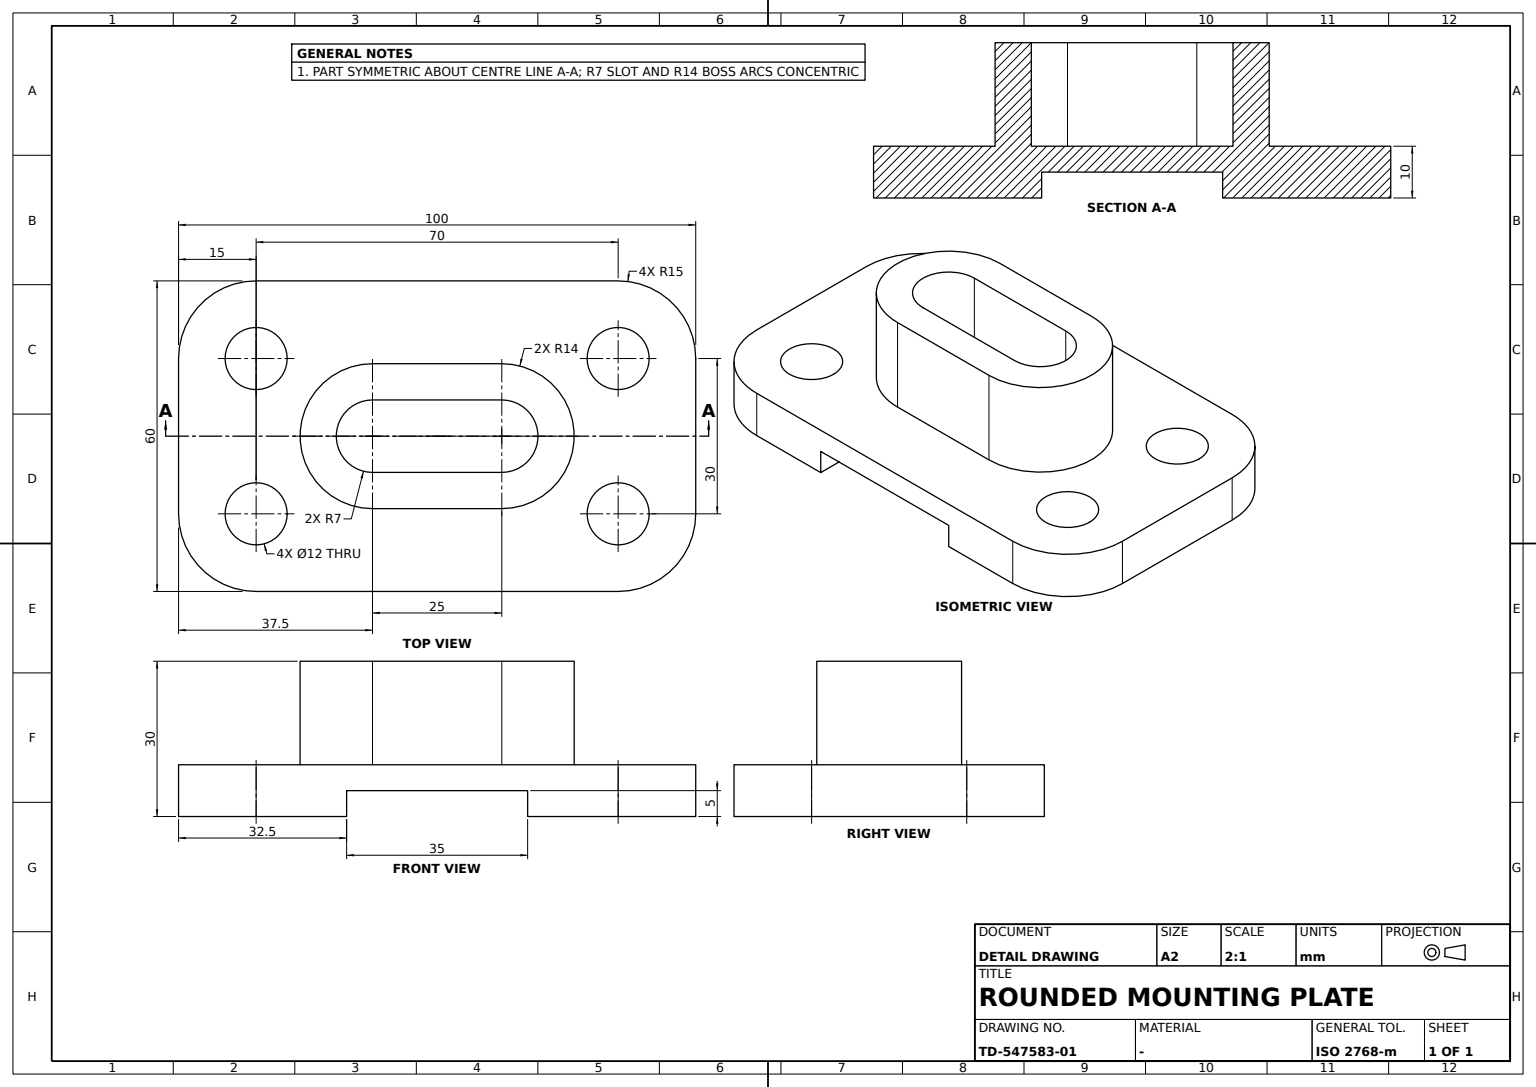
ISO-10303-21;
HEADER;
FILE_DESCRIPTION((''),'2;1');
FILE_NAME('','',(''),(''),'','','');
FILE_SCHEMA(('AUTOMOTIVE_DESIGN'));
ENDSEC;
DATA;
#1=APPLICATION_CONTEXT('');
#2=PRODUCT_CONTEXT('',#1,'mechanical');
#3=PRODUCT('','','',(#2));
#4=PRODUCT_DEFINITION_FORMATION('','',#3);
#5=PRODUCT_DEFINITION_CONTEXT('',#1,'design');
#6=PRODUCT_DEFINITION('','',#4,#5);
#7=PRODUCT_DEFINITION_SHAPE('','',#6);
#8=(LENGTH_UNIT()NAMED_UNIT(*)SI_UNIT(.MILLI.,.METRE.));
#9=(NAMED_UNIT(*)PLANE_ANGLE_UNIT()SI_UNIT($,.RADIAN.));
#10=(NAMED_UNIT(*)SI_UNIT($,.STERADIAN.)SOLID_ANGLE_UNIT());
#11=UNCERTAINTY_MEASURE_WITH_UNIT(LENGTH_MEASURE(0.005),#8,'distance_accuracy_value','');
#12=(GEOMETRIC_REPRESENTATION_CONTEXT(3)GLOBAL_UNCERTAINTY_ASSIGNED_CONTEXT((#11))GLOBAL_UNIT_ASSIGNED_CONTEXT((#8,#9,#10))REPRESENTATION_CONTEXT('',''));
#13=CARTESIAN_POINT('',(17.5,30.,0.));
#14=VERTEX_POINT('',#13);
#15=CARTESIAN_POINT('',(17.5,-30.,0.));
#16=VERTEX_POINT('',#15);
#17=CARTESIAN_POINT('',(17.5,0.,0.));
#18=DIRECTION('',(0.,-1.,0.));
#19=VECTOR('',#18,1000.);
#20=LINE('',#17,#19);
#21=EDGE_CURVE('',#14,#16,#20,.T.);
#22=ORIENTED_EDGE('',*,*,#21,.T.);
#23=CARTESIAN_POINT('',(17.5,-30.,5.));
#24=VERTEX_POINT('',#23);
#25=DIRECTION('',(0.,0.,1.));
#26=VECTOR('',#25,1000.);
#27=LINE('',#15,#26);
#28=EDGE_CURVE('',#16,#24,#27,.T.);
#29=ORIENTED_EDGE('',*,*,#28,.T.);
#30=CARTESIAN_POINT('',(17.5,30.,5.));
#31=VERTEX_POINT('',#30);
#32=LINE('',#30,#19);
#33=EDGE_CURVE('',#31,#24,#32,.T.);
#34=ORIENTED_EDGE('',*,*,#33,.F.);
#35=DIRECTION('',(0.,0.,-1.));
#36=VECTOR('',#35,1000.);
#37=LINE('',#13,#36);
#38=EDGE_CURVE('',#31,#14,#37,.T.);
#39=ORIENTED_EDGE('',*,*,#38,.T.);
#40=EDGE_LOOP('',(#22,#29,#34,#39));
#41=FACE_BOUND('',#40,.T.);
#42=DIRECTION('',(-1.,0.,0.));
#43=AXIS2_PLACEMENT_3D('',#30,#42,#35);
#44=PLANE('',#43);
#45=ADVANCED_FACE('',(#41),#44,.T.);
#46=CARTESIAN_POINT('',(-29.,15.,0.));
#47=VERTEX_POINT('',#46);
#48=CARTESIAN_POINT('',(-35.,15.,0.));
#49=DIRECTION('',(1.,0.,0.));
#50=AXIS2_PLACEMENT_3D('',#48,#25,#49);
#51=CIRCLE('',#50,6.);
#52=EDGE_CURVE('',#47,#47,#51,.T.);
#53=ORIENTED_EDGE('',*,*,#52,.T.);
#54=EDGE_LOOP('',(#53));
#55=FACE_BOUND('',#54,.T.);
#56=CARTESIAN_POINT('',(-50.,-15.,0.));
#57=VERTEX_POINT('',#56);
#58=CARTESIAN_POINT('',(-50.,15.,0.));
#59=VERTEX_POINT('',#58);
#60=CARTESIAN_POINT('',(-50.,0.,0.));
#61=DIRECTION('',(0.,1.,0.));
#62=VECTOR('',#61,1000.);
#63=LINE('',#60,#62);
#64=EDGE_CURVE('',#57,#59,#63,.T.);
#65=ORIENTED_EDGE('',*,*,#64,.T.);
#66=CARTESIAN_POINT('',(-35.,30.,0.));
#67=VERTEX_POINT('',#66);
#68=CIRCLE('',#50,15.);
#69=EDGE_CURVE('',#67,#59,#68,.T.);
#70=ORIENTED_EDGE('',*,*,#69,.F.);
#71=CARTESIAN_POINT('',(-17.5,30.,0.));
#72=VERTEX_POINT('',#71);
#73=CARTESIAN_POINT('',(0.,30.,0.));
#74=VECTOR('',#49,1000.);
#75=LINE('',#73,#74);
#76=EDGE_CURVE('',#67,#72,#75,.T.);
#77=ORIENTED_EDGE('',*,*,#76,.T.);
#78=CARTESIAN_POINT('',(-17.5,-30.,0.));
#79=VERTEX_POINT('',#78);
#80=LINE('',#71,#19);
#81=EDGE_CURVE('',#72,#79,#80,.T.);
#82=ORIENTED_EDGE('',*,*,#81,.T.);
#83=CARTESIAN_POINT('',(-35.,-30.,0.));
#84=VERTEX_POINT('',#83);
#85=CARTESIAN_POINT('',(0.,-30.,0.));
#86=VECTOR('',#42,1000.);
#87=LINE('',#85,#86);
#88=EDGE_CURVE('',#79,#84,#87,.T.);
#89=ORIENTED_EDGE('',*,*,#88,.T.);
#90=CARTESIAN_POINT('',(-35.,-15.,0.));
#91=AXIS2_PLACEMENT_3D('',#90,#25,#49);
#92=CIRCLE('',#91,15.);
#93=EDGE_CURVE('',#57,#84,#92,.T.);
#94=ORIENTED_EDGE('',*,*,#93,.F.);
#95=EDGE_LOOP('',(#65,#70,#77,#82,#89,#94));
#96=FACE_BOUND('',#95,.T.);
#97=CARTESIAN_POINT('',(-29.,-15.,0.));
#98=VERTEX_POINT('',#97);
#99=CIRCLE('',#91,6.);
#100=EDGE_CURVE('',#98,#98,#99,.T.);
#101=ORIENTED_EDGE('',*,*,#100,.T.);
#102=EDGE_LOOP('',(#101));
#103=FACE_BOUND('',#102,.T.);
#104=CARTESIAN_POINT('',(0.,0.,0.));
#105=AXIS2_PLACEMENT_3D('',#104,#25,#49);
#106=PLANE('',#105);
#107=ADVANCED_FACE('',(#55,#96,#103),#106,.F.);
#108=ORIENTED_EDGE('',*,*,#100,.F.);
#109=EDGE_LOOP('',(#108));
#110=FACE_BOUND('',#109,.T.);
#111=CARTESIAN_POINT('',(-29.,-15.,10.));
#112=VERTEX_POINT('',#111);
#113=CARTESIAN_POINT('',(-35.,-15.,10.));
#114=AXIS2_PLACEMENT_3D('',#113,#25,#49);
#115=CIRCLE('',#114,6.);
#116=EDGE_CURVE('',#112,#112,#115,.T.);
#117=ORIENTED_EDGE('',*,*,#116,.T.);
#118=EDGE_LOOP('',(#117));
#119=FACE_BOUND('',#118,.T.);
#120=CARTESIAN_POINT('',(-35.,-15.,5.));
#121=AXIS2_PLACEMENT_3D('',#120,#25,#49);
#122=CYLINDRICAL_SURFACE('',#121,6.);
#123=ADVANCED_FACE('',(#110,#119),#122,.F.);
#124=CARTESIAN_POINT('',(12.5,-14.,30.));
#125=VERTEX_POINT('',#124);
#126=CARTESIAN_POINT('',(12.5,14.,30.));
#127=VERTEX_POINT('',#126);
#128=CARTESIAN_POINT('',(12.5,0.,30.));
#129=AXIS2_PLACEMENT_3D('',#128,#25,#49);
#130=CIRCLE('',#129,14.);
#131=EDGE_CURVE('',#125,#127,#130,.T.);
#132=ORIENTED_EDGE('',*,*,#131,.F.);
#133=CARTESIAN_POINT('',(12.5,-14.,10.));
#134=VERTEX_POINT('',#133);
#135=CARTESIAN_POINT('',(12.5,-14.,20.));
#136=LINE('',#135,#26);
#137=EDGE_CURVE('',#134,#125,#136,.T.);
#138=ORIENTED_EDGE('',*,*,#137,.F.);
#139=CARTESIAN_POINT('',(12.5,14.,10.));
#140=VERTEX_POINT('',#139);
#141=CARTESIAN_POINT('',(12.5,0.,10.));
#142=AXIS2_PLACEMENT_3D('',#141,#25,#49);
#143=CIRCLE('',#142,14.);
#144=EDGE_CURVE('',#134,#140,#143,.T.);
#145=ORIENTED_EDGE('',*,*,#144,.T.);
#146=CARTESIAN_POINT('',(12.5,14.,20.));
#147=LINE('',#146,#26);
#148=EDGE_CURVE('',#140,#127,#147,.T.);
#149=ORIENTED_EDGE('',*,*,#148,.T.);
#150=EDGE_LOOP('',(#132,#138,#145,#149));
#151=FACE_BOUND('',#150,.T.);
#152=CARTESIAN_POINT('',(12.5,0.,20.));
#153=AXIS2_PLACEMENT_3D('',#152,#25,#49);
#154=CYLINDRICAL_SURFACE('',#153,14.);
#155=ADVANCED_FACE('',(#151),#154,.T.);
#156=CARTESIAN_POINT('',(50.,15.,10.));
#157=VERTEX_POINT('',#156);
#158=CARTESIAN_POINT('',(50.,-15.,10.));
#159=VERTEX_POINT('',#158);
#160=CARTESIAN_POINT('',(50.,0.,10.));
#161=LINE('',#160,#19);
#162=EDGE_CURVE('',#157,#159,#161,.T.);
#163=ORIENTED_EDGE('',*,*,#162,.T.);
#164=CARTESIAN_POINT('',(50.,-15.,0.));
#165=VERTEX_POINT('',#164);
#166=CARTESIAN_POINT('',(50.,-15.,5.));
#167=LINE('',#166,#26);
#168=EDGE_CURVE('',#165,#159,#167,.T.);
#169=ORIENTED_EDGE('',*,*,#168,.F.);
#170=CARTESIAN_POINT('',(50.,15.,0.));
#171=VERTEX_POINT('',#170);
#172=CARTESIAN_POINT('',(50.,0.,0.));
#173=LINE('',#172,#19);
#174=EDGE_CURVE('',#171,#165,#173,.T.);
#175=ORIENTED_EDGE('',*,*,#174,.F.);
#176=CARTESIAN_POINT('',(50.,15.,5.));
#177=LINE('',#176,#26);
#178=EDGE_CURVE('',#171,#157,#177,.T.);
#179=ORIENTED_EDGE('',*,*,#178,.T.);
#180=EDGE_LOOP('',(#163,#169,#175,#179));
#181=FACE_BOUND('',#180,.T.);
#182=AXIS2_PLACEMENT_3D('',#170,#42,#18);
#183=PLANE('',#182);
#184=ADVANCED_FACE('',(#181),#183,.F.);
#185=CARTESIAN_POINT('',(-29.,15.,10.));
#186=VERTEX_POINT('',#185);
#187=CARTESIAN_POINT('',(-35.,15.,10.));
#188=AXIS2_PLACEMENT_3D('',#187,#25,#49);
#189=CIRCLE('',#188,6.);
#190=EDGE_CURVE('',#186,#186,#189,.T.);
#191=ORIENTED_EDGE('',*,*,#190,.F.);
#192=EDGE_LOOP('',(#191));
#193=FACE_BOUND('',#192,.T.);
#194=ORIENTED_EDGE('',*,*,#116,.F.);
#195=EDGE_LOOP('',(#194));
#196=FACE_BOUND('',#195,.T.);
#197=CARTESIAN_POINT('',(-50.,-15.,10.));
#198=VERTEX_POINT('',#197);
#199=CARTESIAN_POINT('',(-35.,-30.,10.));
#200=VERTEX_POINT('',#199);
#201=CIRCLE('',#114,15.);
#202=EDGE_CURVE('',#198,#200,#201,.T.);
#203=ORIENTED_EDGE('',*,*,#202,.T.);
#204=CARTESIAN_POINT('',(35.,-30.,10.));
#205=VERTEX_POINT('',#204);
#206=CARTESIAN_POINT('',(0.,-30.,10.));
#207=LINE('',#206,#86);
#208=EDGE_CURVE('',#205,#200,#207,.T.);
#209=ORIENTED_EDGE('',*,*,#208,.F.);
#210=CARTESIAN_POINT('',(35.,-15.,10.));
#211=AXIS2_PLACEMENT_3D('',#210,#25,#49);
#212=CIRCLE('',#211,15.);
#213=EDGE_CURVE('',#205,#159,#212,.T.);
#214=ORIENTED_EDGE('',*,*,#213,.T.);
#215=ORIENTED_EDGE('',*,*,#162,.F.);
#216=CARTESIAN_POINT('',(35.,30.,10.));
#217=VERTEX_POINT('',#216);
#218=CARTESIAN_POINT('',(35.,15.,10.));
#219=AXIS2_PLACEMENT_3D('',#218,#25,#49);
#220=CIRCLE('',#219,15.);
#221=EDGE_CURVE('',#157,#217,#220,.T.);
#222=ORIENTED_EDGE('',*,*,#221,.T.);
#223=CARTESIAN_POINT('',(-35.,30.,10.));
#224=VERTEX_POINT('',#223);
#225=CARTESIAN_POINT('',(0.,30.,10.));
#226=LINE('',#225,#74);
#227=EDGE_CURVE('',#224,#217,#226,.T.);
#228=ORIENTED_EDGE('',*,*,#227,.F.);
#229=CARTESIAN_POINT('',(-50.,15.,10.));
#230=VERTEX_POINT('',#229);
#231=CIRCLE('',#188,15.);
#232=EDGE_CURVE('',#224,#230,#231,.T.);
#233=ORIENTED_EDGE('',*,*,#232,.T.);
#234=CARTESIAN_POINT('',(-50.,0.,10.));
#235=LINE('',#234,#62);
#236=EDGE_CURVE('',#198,#230,#235,.T.);
#237=ORIENTED_EDGE('',*,*,#236,.F.);
#238=EDGE_LOOP('',(#203,#209,#214,#215,#222,#228,#233,#237));
#239=FACE_BOUND('',#238,.T.);
#240=CARTESIAN_POINT('',(-12.5,-14.,10.));
#241=VERTEX_POINT('',#240);
#242=CARTESIAN_POINT('',(0.,-14.,10.));
#243=LINE('',#242,#74);
#244=EDGE_CURVE('',#241,#134,#243,.T.);
#245=ORIENTED_EDGE('',*,*,#244,.F.);
#246=CARTESIAN_POINT('',(-12.5,14.,10.));
#247=VERTEX_POINT('',#246);
#248=CARTESIAN_POINT('',(-12.5,0.,10.));
#249=AXIS2_PLACEMENT_3D('',#248,#25,#49);
#250=CIRCLE('',#249,14.);
#251=EDGE_CURVE('',#247,#241,#250,.T.);
#252=ORIENTED_EDGE('',*,*,#251,.F.);
#253=CARTESIAN_POINT('',(0.,14.,10.));
#254=LINE('',#253,#74);
#255=EDGE_CURVE('',#247,#140,#254,.T.);
#256=ORIENTED_EDGE('',*,*,#255,.T.);
#257=ORIENTED_EDGE('',*,*,#144,.F.);
#258=EDGE_LOOP('',(#245,#252,#256,#257));
#259=FACE_BOUND('',#258,.T.);
#260=CARTESIAN_POINT('',(41.,15.,10.));
#261=VERTEX_POINT('',#260);
#262=CIRCLE('',#219,6.);
#263=EDGE_CURVE('',#261,#261,#262,.T.);
#264=ORIENTED_EDGE('',*,*,#263,.F.);
#265=EDGE_LOOP('',(#264));
#266=FACE_BOUND('',#265,.T.);
#267=CARTESIAN_POINT('',(41.,-15.,10.));
#268=VERTEX_POINT('',#267);
#269=CIRCLE('',#211,6.);
#270=EDGE_CURVE('',#268,#268,#269,.T.);
#271=ORIENTED_EDGE('',*,*,#270,.F.);
#272=EDGE_LOOP('',(#271));
#273=FACE_BOUND('',#272,.T.);
#274=CARTESIAN_POINT('',(0.,0.,10.));
#275=AXIS2_PLACEMENT_3D('',#274,#25,#49);
#276=PLANE('',#275);
#277=ADVANCED_FACE('',(#193,#196,#239,#259,#266,#273),#276,.T.);
#278=CARTESIAN_POINT('',(-12.5,-14.,30.));
#279=VERTEX_POINT('',#278);
#280=CARTESIAN_POINT('',(0.,-14.,30.));
#281=LINE('',#280,#74);
#282=EDGE_CURVE('',#279,#125,#281,.T.);
#283=ORIENTED_EDGE('',*,*,#282,.F.);
#284=CARTESIAN_POINT('',(-12.5,-14.,20.));
#285=LINE('',#284,#26);
#286=EDGE_CURVE('',#241,#279,#285,.T.);
#287=ORIENTED_EDGE('',*,*,#286,.F.);
#288=ORIENTED_EDGE('',*,*,#244,.T.);
#289=ORIENTED_EDGE('',*,*,#137,.T.);
#290=EDGE_LOOP('',(#283,#287,#288,#289));
#291=FACE_BOUND('',#290,.T.);
#292=AXIS2_PLACEMENT_3D('',#240,#18,#49);
#293=PLANE('',#292);
#294=ADVANCED_FACE('',(#291),#293,.T.);
#295=ORIENTED_EDGE('',*,*,#251,.T.);
#296=ORIENTED_EDGE('',*,*,#286,.T.);
#297=CARTESIAN_POINT('',(-12.5,14.,30.));
#298=VERTEX_POINT('',#297);
#299=CARTESIAN_POINT('',(-12.5,0.,30.));
#300=AXIS2_PLACEMENT_3D('',#299,#25,#49);
#301=CIRCLE('',#300,14.);
#302=EDGE_CURVE('',#298,#279,#301,.T.);
#303=ORIENTED_EDGE('',*,*,#302,.F.);
#304=CARTESIAN_POINT('',(-12.5,14.,20.));
#305=LINE('',#304,#26);
#306=EDGE_CURVE('',#247,#298,#305,.T.);
#307=ORIENTED_EDGE('',*,*,#306,.F.);
#308=EDGE_LOOP('',(#295,#296,#303,#307));
#309=FACE_BOUND('',#308,.T.);
#310=CARTESIAN_POINT('',(-12.5,0.,20.));
#311=AXIS2_PLACEMENT_3D('',#310,#25,#49);
#312=CYLINDRICAL_SURFACE('',#311,14.);
#313=ADVANCED_FACE('',(#309),#312,.T.);
#314=CARTESIAN_POINT('',(-17.5,-30.,5.));
#315=VERTEX_POINT('',#314);
#316=LINE('',#78,#26);
#317=EDGE_CURVE('',#79,#315,#316,.T.);
#318=ORIENTED_EDGE('',*,*,#317,.F.);
#319=ORIENTED_EDGE('',*,*,#81,.F.);
#320=CARTESIAN_POINT('',(-17.5,30.,5.));
#321=VERTEX_POINT('',#320);
#322=LINE('',#71,#26);
#323=EDGE_CURVE('',#72,#321,#322,.T.);
#324=ORIENTED_EDGE('',*,*,#323,.T.);
#325=LINE('',#320,#19);
#326=EDGE_CURVE('',#321,#315,#325,.T.);
#327=ORIENTED_EDGE('',*,*,#326,.T.);
#328=EDGE_LOOP('',(#318,#319,#324,#327));
#329=FACE_BOUND('',#328,.T.);
#330=AXIS2_PLACEMENT_3D('',#71,#49,#25);
#331=PLANE('',#330);
#332=ADVANCED_FACE('',(#329),#331,.T.);
#333=ORIENTED_EDGE('',*,*,#190,.T.);
#334=EDGE_LOOP('',(#333));
#335=FACE_BOUND('',#334,.T.);
#336=ORIENTED_EDGE('',*,*,#52,.F.);
#337=EDGE_LOOP('',(#336));
#338=FACE_BOUND('',#337,.T.);
#339=CARTESIAN_POINT('',(-35.,15.,5.));
#340=AXIS2_PLACEMENT_3D('',#339,#25,#49);
#341=CYLINDRICAL_SURFACE('',#340,6.);
#342=ADVANCED_FACE('',(#335,#338),#341,.F.);
#343=CARTESIAN_POINT('',(41.,-15.,0.));
#344=VERTEX_POINT('',#343);
#345=CARTESIAN_POINT('',(35.,-15.,0.));
#346=AXIS2_PLACEMENT_3D('',#345,#25,#49);
#347=CIRCLE('',#346,6.);
#348=EDGE_CURVE('',#344,#344,#347,.T.);
#349=ORIENTED_EDGE('',*,*,#348,.F.);
#350=EDGE_LOOP('',(#349));
#351=FACE_BOUND('',#350,.T.);
#352=ORIENTED_EDGE('',*,*,#270,.T.);
#353=EDGE_LOOP('',(#352));
#354=FACE_BOUND('',#353,.T.);
#355=CARTESIAN_POINT('',(35.,-15.,5.));
#356=AXIS2_PLACEMENT_3D('',#355,#25,#49);
#357=CYLINDRICAL_SURFACE('',#356,6.);
#358=ADVANCED_FACE('',(#351,#354),#357,.F.);
#359=CARTESIAN_POINT('',(-35.,30.,5.));
#360=LINE('',#359,#74);
#361=EDGE_CURVE('',#321,#31,#360,.T.);
#362=ORIENTED_EDGE('',*,*,#361,.T.);
#363=ORIENTED_EDGE('',*,*,#33,.T.);
#364=LINE('',#314,#74);
#365=EDGE_CURVE('',#315,#24,#364,.T.);
#366=ORIENTED_EDGE('',*,*,#365,.F.);
#367=ORIENTED_EDGE('',*,*,#326,.F.);
#368=EDGE_LOOP('',(#362,#363,#366,#367));
#369=FACE_BOUND('',#368,.T.);
#370=AXIS2_PLACEMENT_3D('',#320,#35,#49);
#371=PLANE('',#370);
#372=ADVANCED_FACE('',(#369),#371,.T.);
#373=CARTESIAN_POINT('',(-12.5,-7.,30.));
#374=VERTEX_POINT('',#373);
#375=CARTESIAN_POINT('',(12.5,-7.,30.));
#376=VERTEX_POINT('',#375);
#377=CARTESIAN_POINT('',(0.,-7.,30.));
#378=LINE('',#377,#74);
#379=EDGE_CURVE('',#374,#376,#378,.T.);
#380=ORIENTED_EDGE('',*,*,#379,.F.);
#381=CARTESIAN_POINT('',(-12.5,7.,30.));
#382=VERTEX_POINT('',#381);
#383=CIRCLE('',#300,7.);
#384=EDGE_CURVE('',#382,#374,#383,.T.);
#385=ORIENTED_EDGE('',*,*,#384,.F.);
#386=CARTESIAN_POINT('',(12.5,7.,30.));
#387=VERTEX_POINT('',#386);
#388=CARTESIAN_POINT('',(0.,7.,30.));
#389=LINE('',#388,#74);
#390=EDGE_CURVE('',#382,#387,#389,.T.);
#391=ORIENTED_EDGE('',*,*,#390,.T.);
#392=CIRCLE('',#129,7.);
#393=EDGE_CURVE('',#376,#387,#392,.T.);
#394=ORIENTED_EDGE('',*,*,#393,.F.);
#395=EDGE_LOOP('',(#380,#385,#391,#394));
#396=FACE_BOUND('',#395,.T.);
#397=ORIENTED_EDGE('',*,*,#131,.T.);
#398=CARTESIAN_POINT('',(0.,14.,30.));
#399=LINE('',#398,#74);
#400=EDGE_CURVE('',#298,#127,#399,.T.);
#401=ORIENTED_EDGE('',*,*,#400,.F.);
#402=ORIENTED_EDGE('',*,*,#302,.T.);
#403=ORIENTED_EDGE('',*,*,#282,.T.);
#404=EDGE_LOOP('',(#397,#401,#402,#403));
#405=FACE_BOUND('',#404,.T.);
#406=CARTESIAN_POINT('',(0.,0.,30.));
#407=AXIS2_PLACEMENT_3D('',#406,#25,#49);
#408=PLANE('',#407);
#409=ADVANCED_FACE('',(#396,#405),#408,.T.);
#410=CARTESIAN_POINT('',(-35.,-30.,5.));
#411=LINE('',#410,#26);
#412=EDGE_CURVE('',#84,#200,#411,.T.);
#413=ORIENTED_EDGE('',*,*,#412,.T.);
#414=ORIENTED_EDGE('',*,*,#202,.F.);
#415=CARTESIAN_POINT('',(-50.,-15.,5.));
#416=LINE('',#415,#26);
#417=EDGE_CURVE('',#57,#198,#416,.T.);
#418=ORIENTED_EDGE('',*,*,#417,.F.);
#419=ORIENTED_EDGE('',*,*,#93,.T.);
#420=EDGE_LOOP('',(#413,#414,#418,#419));
#421=FACE_BOUND('',#420,.T.);
#422=CYLINDRICAL_SURFACE('',#121,15.);
#423=ADVANCED_FACE('',(#421),#422,.T.);
#424=CARTESIAN_POINT('',(12.5,-7.,10.));
#425=VERTEX_POINT('',#424);
#426=CARTESIAN_POINT('',(12.5,7.,10.));
#427=VERTEX_POINT('',#426);
#428=CIRCLE('',#142,7.);
#429=EDGE_CURVE('',#425,#427,#428,.T.);
#430=ORIENTED_EDGE('',*,*,#429,.T.);
#431=CARTESIAN_POINT('',(-12.5,7.,10.));
#432=VERTEX_POINT('',#431);
#433=CARTESIAN_POINT('',(0.,7.,10.));
#434=LINE('',#433,#74);
#435=EDGE_CURVE('',#432,#427,#434,.T.);
#436=ORIENTED_EDGE('',*,*,#435,.F.);
#437=CARTESIAN_POINT('',(-12.5,-7.,10.));
#438=VERTEX_POINT('',#437);
#439=CIRCLE('',#249,7.);
#440=EDGE_CURVE('',#432,#438,#439,.T.);
#441=ORIENTED_EDGE('',*,*,#440,.T.);
#442=CARTESIAN_POINT('',(0.,-7.,10.));
#443=LINE('',#442,#74);
#444=EDGE_CURVE('',#438,#425,#443,.T.);
#445=ORIENTED_EDGE('',*,*,#444,.T.);
#446=EDGE_LOOP('',(#430,#436,#441,#445));
#447=FACE_BOUND('',#446,.T.);
#448=ADVANCED_FACE('',(#447),#276,.T.);
#449=ORIENTED_EDGE('',*,*,#236,.T.);
#450=CARTESIAN_POINT('',(-50.,15.,5.));
#451=LINE('',#450,#26);
#452=EDGE_CURVE('',#59,#230,#451,.T.);
#453=ORIENTED_EDGE('',*,*,#452,.F.);
#454=ORIENTED_EDGE('',*,*,#64,.F.);
#455=ORIENTED_EDGE('',*,*,#417,.T.);
#456=EDGE_LOOP('',(#449,#453,#454,#455));
#457=FACE_BOUND('',#456,.T.);
#458=AXIS2_PLACEMENT_3D('',#56,#49,#61);
#459=PLANE('',#458);
#460=ADVANCED_FACE('',(#457),#459,.F.);
#461=CARTESIAN_POINT('',(35.,30.,0.));
#462=VERTEX_POINT('',#461);
#463=CARTESIAN_POINT('',(35.,15.,0.));
#464=AXIS2_PLACEMENT_3D('',#463,#25,#49);
#465=CIRCLE('',#464,15.);
#466=EDGE_CURVE('',#171,#462,#465,.T.);
#467=ORIENTED_EDGE('',*,*,#466,.T.);
#468=CARTESIAN_POINT('',(35.,30.,5.));
#469=LINE('',#468,#26);
#470=EDGE_CURVE('',#462,#217,#469,.T.);
#471=ORIENTED_EDGE('',*,*,#470,.T.);
#472=ORIENTED_EDGE('',*,*,#221,.F.);
#473=ORIENTED_EDGE('',*,*,#178,.F.);
#474=EDGE_LOOP('',(#467,#471,#472,#473));
#475=FACE_BOUND('',#474,.T.);
#476=CARTESIAN_POINT('',(35.,15.,5.));
#477=AXIS2_PLACEMENT_3D('',#476,#25,#49);
#478=CYLINDRICAL_SURFACE('',#477,15.);
#479=ADVANCED_FACE('',(#475),#478,.T.);
#480=LINE('',#359,#26);
#481=EDGE_CURVE('',#67,#224,#480,.T.);
#482=ORIENTED_EDGE('',*,*,#481,.T.);
#483=ORIENTED_EDGE('',*,*,#227,.T.);
#484=ORIENTED_EDGE('',*,*,#470,.F.);
#485=EDGE_CURVE('',#14,#462,#75,.T.);
#486=ORIENTED_EDGE('',*,*,#485,.F.);
#487=ORIENTED_EDGE('',*,*,#38,.F.);
#488=ORIENTED_EDGE('',*,*,#361,.F.);
#489=ORIENTED_EDGE('',*,*,#323,.F.);
#490=ORIENTED_EDGE('',*,*,#76,.F.);
#491=EDGE_LOOP('',(#482,#483,#484,#486,#487,#488,#489,#490));
#492=FACE_BOUND('',#491,.T.);
#493=AXIS2_PLACEMENT_3D('',#66,#18,#49);
#494=PLANE('',#493);
#495=ADVANCED_FACE('',(#492),#494,.F.);
#496=CARTESIAN_POINT('',(41.,15.,0.));
#497=VERTEX_POINT('',#496);
#498=CIRCLE('',#464,6.);
#499=EDGE_CURVE('',#497,#497,#498,.T.);
#500=ORIENTED_EDGE('',*,*,#499,.F.);
#501=EDGE_LOOP('',(#500));
#502=FACE_BOUND('',#501,.T.);
#503=ORIENTED_EDGE('',*,*,#263,.T.);
#504=EDGE_LOOP('',(#503));
#505=FACE_BOUND('',#504,.T.);
#506=CYLINDRICAL_SURFACE('',#477,6.);
#507=ADVANCED_FACE('',(#502,#505),#506,.F.);
#508=CARTESIAN_POINT('',(35.,-30.,0.));
#509=VERTEX_POINT('',#508);
#510=CARTESIAN_POINT('',(35.,-30.,5.));
#511=LINE('',#510,#26);
#512=EDGE_CURVE('',#509,#205,#511,.T.);
#513=ORIENTED_EDGE('',*,*,#512,.F.);
#514=CIRCLE('',#346,15.);
#515=EDGE_CURVE('',#509,#165,#514,.T.);
#516=ORIENTED_EDGE('',*,*,#515,.T.);
#517=ORIENTED_EDGE('',*,*,#168,.T.);
#518=ORIENTED_EDGE('',*,*,#213,.F.);
#519=EDGE_LOOP('',(#513,#516,#517,#518));
#520=FACE_BOUND('',#519,.T.);
#521=CYLINDRICAL_SURFACE('',#356,15.);
#522=ADVANCED_FACE('',(#520),#521,.T.);
#523=ORIENTED_EDGE('',*,*,#306,.T.);
#524=ORIENTED_EDGE('',*,*,#400,.T.);
#525=ORIENTED_EDGE('',*,*,#148,.F.);
#526=ORIENTED_EDGE('',*,*,#255,.F.);
#527=EDGE_LOOP('',(#523,#524,#525,#526));
#528=FACE_BOUND('',#527,.T.);
#529=AXIS2_PLACEMENT_3D('',#246,#18,#49);
#530=PLANE('',#529);
#531=ADVANCED_FACE('',(#528),#530,.F.);
#532=EDGE_CURVE('',#509,#16,#87,.T.);
#533=ORIENTED_EDGE('',*,*,#532,.F.);
#534=ORIENTED_EDGE('',*,*,#512,.T.);
#535=ORIENTED_EDGE('',*,*,#208,.T.);
#536=ORIENTED_EDGE('',*,*,#412,.F.);
#537=ORIENTED_EDGE('',*,*,#88,.F.);
#538=ORIENTED_EDGE('',*,*,#317,.T.);
#539=ORIENTED_EDGE('',*,*,#365,.T.);
#540=ORIENTED_EDGE('',*,*,#28,.F.);
#541=EDGE_LOOP('',(#533,#534,#535,#536,#537,#538,#539,#540));
#542=FACE_BOUND('',#541,.T.);
#543=AXIS2_PLACEMENT_3D('',#508,#61,#42);
#544=PLANE('',#543);
#545=ADVANCED_FACE('',(#542),#544,.F.);
#546=CARTESIAN_POINT('',(12.5,7.,20.));
#547=LINE('',#546,#26);
#548=EDGE_CURVE('',#427,#387,#547,.T.);
#549=ORIENTED_EDGE('',*,*,#548,.F.);
#550=ORIENTED_EDGE('',*,*,#429,.F.);
#551=CARTESIAN_POINT('',(12.5,-7.,20.));
#552=LINE('',#551,#26);
#553=EDGE_CURVE('',#425,#376,#552,.T.);
#554=ORIENTED_EDGE('',*,*,#553,.T.);
#555=ORIENTED_EDGE('',*,*,#393,.T.);
#556=EDGE_LOOP('',(#549,#550,#554,#555));
#557=FACE_BOUND('',#556,.T.);
#558=CYLINDRICAL_SURFACE('',#153,7.);
#559=ADVANCED_FACE('',(#557),#558,.F.);
#560=ORIENTED_EDGE('',*,*,#348,.T.);
#561=EDGE_LOOP('',(#560));
#562=FACE_BOUND('',#561,.T.);
#563=ORIENTED_EDGE('',*,*,#174,.T.);
#564=ORIENTED_EDGE('',*,*,#515,.F.);
#565=ORIENTED_EDGE('',*,*,#532,.T.);
#566=ORIENTED_EDGE('',*,*,#21,.F.);
#567=ORIENTED_EDGE('',*,*,#485,.T.);
#568=ORIENTED_EDGE('',*,*,#466,.F.);
#569=EDGE_LOOP('',(#563,#564,#565,#566,#567,#568));
#570=FACE_BOUND('',#569,.T.);
#571=ORIENTED_EDGE('',*,*,#499,.T.);
#572=EDGE_LOOP('',(#571));
#573=FACE_BOUND('',#572,.T.);
#574=ADVANCED_FACE('',(#562,#570,#573),#106,.F.);
#575=CARTESIAN_POINT('',(-12.5,-7.,20.));
#576=LINE('',#575,#26);
#577=EDGE_CURVE('',#438,#374,#576,.T.);
#578=ORIENTED_EDGE('',*,*,#577,.T.);
#579=ORIENTED_EDGE('',*,*,#379,.T.);
#580=ORIENTED_EDGE('',*,*,#553,.F.);
#581=ORIENTED_EDGE('',*,*,#444,.F.);
#582=EDGE_LOOP('',(#578,#579,#580,#581));
#583=FACE_BOUND('',#582,.T.);
#584=AXIS2_PLACEMENT_3D('',#437,#18,#49);
#585=PLANE('',#584);
#586=ADVANCED_FACE('',(#583),#585,.F.);
#587=ORIENTED_EDGE('',*,*,#577,.F.);
#588=ORIENTED_EDGE('',*,*,#440,.F.);
#589=CARTESIAN_POINT('',(-12.5,7.,20.));
#590=LINE('',#589,#26);
#591=EDGE_CURVE('',#432,#382,#590,.T.);
#592=ORIENTED_EDGE('',*,*,#591,.T.);
#593=ORIENTED_EDGE('',*,*,#384,.T.);
#594=EDGE_LOOP('',(#587,#588,#592,#593));
#595=FACE_BOUND('',#594,.T.);
#596=CYLINDRICAL_SURFACE('',#311,7.);
#597=ADVANCED_FACE('',(#595),#596,.F.);
#598=ORIENTED_EDGE('',*,*,#232,.F.);
#599=ORIENTED_EDGE('',*,*,#481,.F.);
#600=ORIENTED_EDGE('',*,*,#69,.T.);
#601=ORIENTED_EDGE('',*,*,#452,.T.);
#602=EDGE_LOOP('',(#598,#599,#600,#601));
#603=FACE_BOUND('',#602,.T.);
#604=CYLINDRICAL_SURFACE('',#340,15.);
#605=ADVANCED_FACE('',(#603),#604,.T.);
#606=ORIENTED_EDGE('',*,*,#435,.T.);
#607=ORIENTED_EDGE('',*,*,#548,.T.);
#608=ORIENTED_EDGE('',*,*,#390,.F.);
#609=ORIENTED_EDGE('',*,*,#591,.F.);
#610=EDGE_LOOP('',(#606,#607,#608,#609));
#611=FACE_BOUND('',#610,.T.);
#612=AXIS2_PLACEMENT_3D('',#431,#18,#49);
#613=PLANE('',#612);
#614=ADVANCED_FACE('',(#611),#613,.T.);
#615=CLOSED_SHELL('',(#45,#107,#123,#155,#184,#277,#294,#313,#332,#342,#358,#372,#409,#423,#448,#460,#479,#495,#507,#522,#531,#545,#559,#574,#586,#597,#605,#614));
#616=MANIFOLD_SOLID_BREP('',#615);
#617=ADVANCED_BREP_SHAPE_REPRESENTATION('',(#616),#12);
#618=SHAPE_DEFINITION_REPRESENTATION(#7,#617);
ENDSEC;
END-ISO-10303-21;
